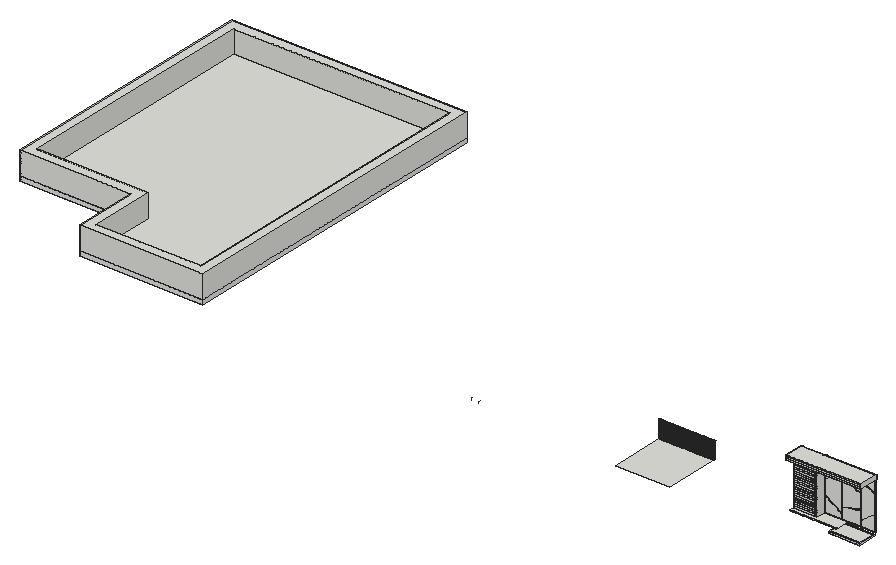
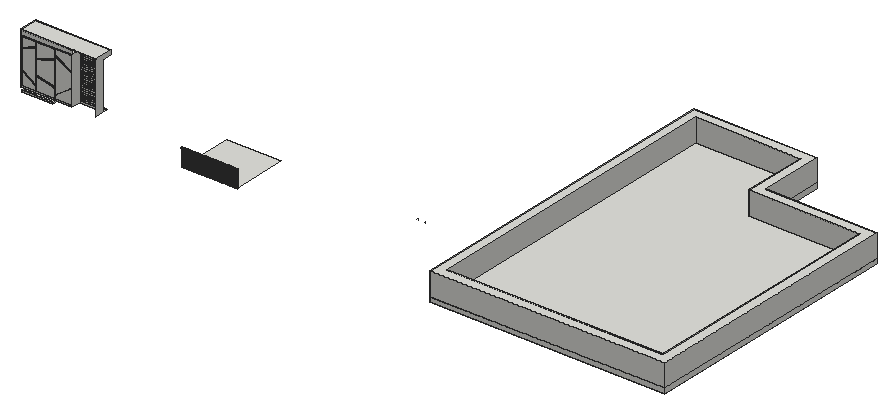
# SketchUp Ruby script. Lengths in inches.
U = 1.inch
M = Sketchup.active_model
def pt(a) = Geom::Point3d.new(a.map { |v| v * U })
def face(e, loops, mat)
  f = e.add_face(loops[0].map { |a| pt(a) })
  loops[1..].each { |l| e.add_face(l.map { |a| pt(a) }).erase! }
  f.material = f.back_material = mat if mat
  f
end
# faces: each face lists its corners as indices into pts; further lists are holes
def faces(e, pts, list, mat = nil) = list.each { |f| face(e, (f[0].is_a?(Array) ? f : [f]).map { |l| l.map { |i| pts[i] } }, mat) }
# xy, xz, yz: faces in a plane at the given z, y or x. An outline is a flat list of corners, or four numbers for a rectangle; further outlines are holes
def ring(l) = l.size == 4 ? [[l[0], l[1]], [l[2], l[1]], [l[2], l[3]], [l[0], l[3]]] : l.each_slice(2).to_a
def flat(e, list, mat, &to3) = list.each { |f| face(e, (f[0].is_a?(Array) ? f : [f]).map { |l| ring(l).map { |u, v| to3.(u, v) } }, mat) }
def xy(e, z, list, mat = nil) = flat(e, list, mat) { |x, y| [x, y, z] }
def xz(e, y, list, mat = nil) = flat(e, list, mat) { |x, z| [x, y, z] }
def yz(e, x, list, mat = nil) = flat(e, list, mat) { |y, z| [x, y, z] }
def lines(e, pts, list) = list.each { |a, b| e.add_line(pt(pts[a]), pt(pts[b])) }
# prism: a flat outline (further loops are holes) pulled along v
def prism(e, loops, v, mat = nil)
  f = face(e, loops, mat); d = Geom::Vector3d.new(v.map { |x| x * U })
  f.pushpull(f.normal.samedirection?(d) ? d.length : -d.length)
end
def box(e, o, s, mat = nil) = prism(e, [[o, [o[0] + s[0], o[1], o[2]], [o[0] + s[0], o[1] + s[1], o[2]], [o[0], o[1] + s[1], o[2]]]], [0, 0, s[2]], mat)
def at(x, y, z, deg = 0) = Geom::Transformation.translation(pt([x, y, z])) * Geom::Transformation.rotation(ORIGIN, Z_AXIS, deg.degrees)
def axes(o, x, y, z) = Geom::Transformation.new([*x, 0, *y, 0, *z, 0, *pt(o).to_a, 1])
def part(name) = M.definitions.add(name)
# library, detail: a bought-in or finely detailed component or shape, given as its bounding box
def library(name, o, s) = part(name).tap { |d| box(d.entities, o, s) }
def detail(e, o, s) = box(e.add_group.entities, o, s)
def put(e, d, t, mat = nil) = e.add_instance(d, t).tap { |i| i.material = mat if mat }
def group(e, t, mat = nil) = e.add_group.tap { |g| g.transformation = t; g.material = mat if mat }.entities
root = M.entities
xy(root,13.08,[[971.17,172.59,1011.17,196.59]])
xy(root,14,[[719.98,146.23,789.98,216.23],[718.98,216.23,719.98,216.73],[719.98,216.23,720.98,216.73],[721.48,216.23,722.48,216.73],[722.48,216.23,723.48,216.73],
  [723.98,216.23,724.98,216.73],[724.98,216.23,725.98,216.73],[726.48,216.23,727.48,216.73],[727.48,216.23,728.48,216.73],[728.98,216.23,729.98,216.73],
  [729.98,216.23,730.98,216.73],[731.48,216.23,732.48,216.73],[732.48,216.23,733.48,216.73],[733.98,216.23,734.98,216.73],[734.98,216.23,735.98,216.73],
  [736.48,216.23,737.48,216.73],[737.48,216.23,738.48,216.73],[738.98,216.23,739.98,216.73],[739.98,216.23,740.98,216.73],[741.48,216.23,742.48,216.73],
  [742.48,216.23,743.48,216.73],[743.98,216.23,744.98,216.73],[744.98,216.23,745.98,216.73],[746.48,216.23,747.48,216.73],[747.48,216.23,748.48,216.73],
  [748.98,216.23,749.98,216.73],[749.98,216.23,750.98,216.73],[751.48,216.23,752.48,216.73],[752.48,216.23,753.48,216.73],[753.98,216.23,754.98,216.73],
  [754.98,216.23,755.98,216.73],[756.48,216.23,757.48,216.73],[757.48,216.23,758.48,216.73],[758.98,216.23,759.98,216.73],[759.98,216.23,760.98,216.73],
  [761.48,216.23,762.48,216.73],[762.48,216.23,763.48,216.73],[763.98,216.23,764.98,216.73],[764.98,216.23,765.98,216.73],[766.48,216.23,767.48,216.73],
  [767.48,216.23,768.48,216.73],[768.98,216.23,769.98,216.73],[769.98,216.23,770.98,216.73],[771.48,216.23,772.48,216.73],[772.48,216.23,773.48,216.73],
  [773.98,216.23,774.98,216.73],[774.98,216.23,775.98,216.73],[776.48,216.23,777.48,216.73],[777.48,216.23,778.48,216.73],[778.98,216.23,779.98,216.73],
  [779.98,216.23,780.98,216.73],[781.48,216.23,782.48,216.73],[782.48,216.23,783.48,216.73],[783.98,216.23,784.98,216.73],[784.98,216.23,785.98,216.73],
  [786.48,216.23,787.48,216.73],[787.48,216.23,788.48,216.73],[788.98,216.23,789.98,216.73],[789.98,216.23,790.98,216.73]])
xy(root,15.08,[[[971.17,172.59,1011.17,196.59],[972.05,173.47,1010.3,195.72]],[972.05,173.47,1010.3,195.72]])
xy(root,18,[[917.17,178.09,919.17,178.59],[919.67,178.09,921.67,178.59],[922.17,178.09,924.17,178.59],[924.67,178.09,926.67,178.59],[927.17,178.09,929.17,178.59],
  [929.67,178.09,931.67,178.59],[932.17,178.09,934.17,178.59],[934.67,178.09,936.67,178.59],[937.17,178.09,939.17,178.59],[939.67,178.09,941.67,178.59],
  [942.17,178.09,944.17,178.59],[944.67,178.09,946.67,178.59],[947.17,178.09,949.17,178.59],[949.67,178.09,951.67,178.59],[952.17,178.09,954.17,178.59],
  [954.67,178.09,956.67,178.59],[957.17,178.09,959.17,178.59],[959.67,178.09,961.67,178.59],[962.17,178.09,964.17,178.59],[964.67,178.09,966.67,178.59],
  [967.17,178.09,969.17,178.59],[969.67,178.09,971.67,178.59],[972.17,178.09,974.17,178.59],[974.67,178.09,976.67,178.59],[917.17,178.59,977.17,178.59,977.17,196.09,947.17,196.09,947.17,184.09,917.17,184.09],
  [917.17,184.09,947.17,184.59]])
xy(root,19,[[994.17,195.59,1012.17,196.09],[948.17,195.72,969.17,196.09],[969.67,195.72,977.17,196.09],[977.17,195.72,993.67,196.09]])
xy(root,20,[[917.17,184.09,947.17,184.59]])
xy(root,20.5,[[917.17,184.09,947.17,184.59]])
xy(root,22.5,[[917.17,184.09,947.17,184.59]])
xy(root,23,[[917.17,184.09,947.17,184.59]])
xy(root,25,[[917.17,184.09,947.17,184.59]])
xy(root,25.5,[[917.17,184.09,947.17,184.59]])
xy(root,27.5,[[917.17,184.09,947.17,184.59]])
xy(root,28,[[917.17,184.09,947.17,184.59]])
xy(root,30,[[917.17,184.09,947.17,184.59]])
xy(root,30.5,[[917.17,184.09,947.17,184.59]])
xy(root,32.5,[[917.17,184.09,947.17,184.59]])
xy(root,33,[[917.17,184.09,947.17,184.59]])
xy(root,35,[[917.17,184.09,947.17,184.59]])
xy(root,35.5,[[917.17,184.09,947.17,184.59]])
xy(root,36,[[718.98,216.23,720.98,216.73],[721.48,216.23,723.48,216.73],[723.98,216.23,725.98,216.73],[726.48,216.23,728.48,216.73],[728.98,216.23,730.98,216.73],
  [731.48,216.23,733.48,216.73],[733.98,216.23,735.98,216.73],[736.48,216.23,738.48,216.73],[738.98,216.23,740.98,216.73],[741.48,216.23,743.48,216.73],
  [743.98,216.23,745.98,216.73],[746.48,216.23,748.48,216.73],[748.98,216.23,750.98,216.73],[751.48,216.23,753.48,216.73],[753.98,216.23,755.98,216.73],
  [756.48,216.23,758.48,216.73],[758.98,216.23,760.98,216.73],[761.48,216.23,763.48,216.73],[763.98,216.23,765.98,216.73],[766.48,216.23,768.48,216.73],
  [768.98,216.23,770.98,216.73],[771.48,216.23,773.48,216.73],[773.98,216.23,775.98,216.73],[776.48,216.23,778.48,216.73],[778.98,216.23,780.98,216.73],
  [781.48,216.23,783.48,216.73],[783.98,216.23,785.98,216.73],[786.48,216.23,788.48,216.73],[788.98,216.23,790.98,216.73],[718.98,216.73,790.98,217.23]])
xy(root,37.5,[[917.17,184.09,947.17,184.59]])
xy(root,38,[[917.17,184.09,947.17,184.59]])
xy(root,40,[[917.17,184.09,947.17,184.59]])
xy(root,40.5,[[917.17,184.09,947.17,184.59]])
xy(root,42.5,[[917.17,184.09,947.17,184.59]])
xy(root,43,[[917.17,184.09,947.17,184.59]])
xy(root,45,[[917.17,184.09,947.17,184.59]])
xy(root,45.5,[[917.17,184.09,947.17,184.59]])
xy(root,47.5,[[917.17,184.09,947.17,184.59]])
xy(root,48,[[917.17,184.09,947.17,184.59]])
xy(root,50,[[917.17,184.09,947.17,184.59]])
xy(root,50.5,[[917.17,184.09,947.17,184.59]])
xy(root,52.5,[[917.17,184.09,947.17,184.59]])
xy(root,53,[[917.17,184.09,947.17,184.59]])
xy(root,55,[[917.17,184.09,947.17,184.59]])
xy(root,55.5,[[917.17,184.09,947.17,184.59]])
xy(root,57.5,[[917.17,184.09,947.17,184.59]])
xy(root,58,[[917.17,184.09,947.17,184.59]])
xy(root,60,[[917.17,184.09,947.17,184.59]])
xy(root,60.5,[[917.17,184.09,947.17,184.59]])
xy(root,62.5,[[917.17,184.09,947.17,184.59]])
xy(root,63,[[917.17,184.09,947.17,184.59]])
xy(root,65,[[917.17,184.09,947.17,184.59]])
xy(root,65.5,[[917.17,184.09,947.17,184.59]])
xy(root,67.5,[[917.17,184.09,947.17,184.59]])
xy(root,68,[[917.17,184.09,947.17,184.59]])
xy(root,70,[[917.17,184.09,947.17,184.59]])
xy(root,70.5,[[917.17,184.09,947.17,184.59]])
xy(root,72.5,[[917.17,184.09,947.17,184.59]])
xy(root,73,[[917.17,184.09,947.17,184.59]])
xy(root,75,[[917.17,184.09,947.17,184.59]])
xy(root,75.5,[[917.17,184.09,947.17,184.59]])
xy(root,77,[[994.17,195.59,1012.17,196.09],[948.17,195.72,969.17,196.09],[969.67,195.72,993.67,196.09]])
xy(root,77.5,[[917.17,184.09,947.17,184.59]])
xy(root,78,[[917.17,172.59,917.17,184.59,947.17,184.59,947.17,196.09,1013.17,196.09,1011.17,172.59],[1011.17,172.59,1013.17,196.09,1013.17,172.59]])
xy(root,84,[[917.17,172.59,1013.17,196.09],[917.17,196.09,947.17,196.59],[947.17,196.09,1013.17,196.59]])
xz(root,172.59,[[[971.17,13.08,1011.17,15.08],[971.67,13.58,1010.67,14.58]],[971.67,13.58,1010.67,14.58],[[917.17,78,1013.17,84],[918.17,79,1012.17,83]],[918.17,79,1012.17,83]])
xz(root,184.09,[[917.17,18,947.17,20],[917.17,20.5,947.17,22.5],[917.17,23,947.17,25],[917.17,25.5,947.17,27.5],[917.17,28,947.17,30],
  [917.17,30.5,947.17,32.5],[917.17,33,947.17,35],[917.17,35.5,947.17,37.5],[917.17,38,947.17,40],[917.17,40.5,947.17,42.5],
  [917.17,43,947.17,45],[917.17,45.5,947.17,47.5],[917.17,48,947.17,50],[917.17,50.5,947.17,52.5],[917.17,53,947.17,55],
  [917.17,55.5,947.17,57.5],[917.17,58,947.17,60],[917.17,60.5,947.17,62.5],[917.17,63,947.17,65],[917.17,65.5,947.17,67.5],
  [917.17,68,947.17,70],[917.17,70.5,947.17,72.5],[917.17,73,947.17,75],[917.17,75.5,947.17,77.5]])
xz(root,184.59,[[917.17,18,947.17,20],[917.17,20,947.17,20.5],[917.17,20.5,947.17,22.5],[917.17,22.5,947.17,23],[917.17,23,947.17,25],
  [917.17,25,947.17,25.5],[917.17,25.5,947.17,27.5],[917.17,27.5,947.17,28],[917.17,28,947.17,30],[917.17,30,947.17,30.5],
  [917.17,30.5,947.17,32.5],[917.17,32.5,947.17,33],[917.17,33,947.17,35],[917.17,35,947.17,35.5],[917.17,35.5,947.17,37.5],
  [917.17,37.5,947.17,38],[917.17,38,947.17,40],[917.17,40,947.17,40.5],[917.17,40.5,947.17,42.5],[917.17,42.5,947.17,43],
  [917.17,43,947.17,45],[917.17,45,947.17,45.5],[917.17,45.5,947.17,47.5],[917.17,47.5,947.17,48],[917.17,48,947.17,50],
  [917.17,50,947.17,50.5],[917.17,50.5,947.17,52.5],[917.17,52.5,947.17,53],[917.17,53,947.17,55],[917.17,55,947.17,55.5],
  [917.17,55.5,947.17,57.5],[917.17,57.5,947.17,58],[917.17,58,947.17,60],[917.17,60,947.17,60.5],[917.17,60.5,947.17,62.5],
  [917.17,62.5,947.17,63],[917.17,63,947.17,65],[917.17,65,947.17,65.5],[917.17,65.5,947.17,67.5],[917.17,67.5,947.17,68],
  [917.17,68,947.17,70],[917.17,70,947.17,70.5],[917.17,70.5,947.17,72.5],[917.17,72.5,947.17,73],[917.17,73,947.17,75],
  [917.17,75,947.17,75.5],[917.17,75.5,947.17,77.5],[917.17,77.5,947.17,78]])
xz(root,195.59,[[994.17,19,1012.17,19,1012.17,37.79,994.17,25.79],[994.17,26.39,1012.17,38.39,1012.17,62.76,994.17,70.87],[1012.17,63.3125,1012.17,77,994.17,77,994.17,71.42]])
xz(root,195.72,[[948.17,19,969.17,19,969.17,23.8,948.17,38.21],[969.67,19,993.67,19,993.67,37.88,969.67,32.37],[969.17,24.4,969.17,69.42,948.17,56.84,948.17,38.82],[969.67,32.88,993.67,38.39,993.67,55.9,969.67,65.8],[993.67,56.44,993.67,77,969.67,77,969.67,66.34],
  [948.17,57.42,969.17,70.01,969.17,77,948.17,77]])
xz(root,196.09,[[[947.17,18,1013.17,78],[948.17,19,1012.17,77]],[969.17,19,969.67,77],[993.67,19,994.17,77],[969.17,23.8,969.17,24.4,948.17,38.82,948.17,38.21],[994.17,25.79,1012.17,37.79,1012.17,38.39,994.17,26.39],
  [969.67,32.37,993.67,37.88,993.67,38.39,969.67,32.88],[993.67,55.9,993.67,56.44,969.67,66.34,969.67,65.8],[948.17,56.84,969.17,69.42,969.17,70.01,948.17,57.42],[1012.17,62.76,1012.17,63.3125,994.17,71.42,994.17,70.87],[947.17,78,1013.17,84]])
xz(root,196.59,[[971.17,13.08,1011.17,15.08]])
xz(root,216.23,[[718.98,14,720.98,36],[721.48,14,723.48,36],[723.98,14,725.98,36],[726.48,14,728.48,36],[728.98,14,730.98,36],
  [731.48,14,733.48,36],[733.98,14,735.98,36],[736.48,14,738.48,36],[738.98,14,740.98,36],[741.48,14,743.48,36],
  [743.98,14,745.98,36],[746.48,14,748.48,36],[748.98,14,750.98,36],[751.48,14,753.48,36],[753.98,14,755.98,36],
  [756.48,14,758.48,36],[758.98,14,760.98,36],[761.48,14,763.48,36],[763.98,14,765.98,36],[766.48,14,768.48,36],
  [768.98,14,770.98,36],[771.48,14,773.48,36],[773.98,14,775.98,36],[776.48,14,778.48,36],[778.98,14,780.98,36],
  [781.48,14,783.48,36],[783.98,14,785.98,36],[786.48,14,788.48,36],[788.98,14,790.98,36]])
xz(root,216.73,[[718.98,14,720.98,36],[721.48,14,723.48,36],[723.98,14,725.98,36],[726.48,14,728.48,36],[728.98,14,730.98,36],
  [731.48,14,733.48,36],[733.98,14,735.98,36],[736.48,14,738.48,36],[738.98,14,740.98,36],[741.48,14,743.48,36],
  [743.98,14,745.98,36],[746.48,14,748.48,36],[748.98,14,750.98,36],[751.48,14,753.48,36],[753.98,14,755.98,36],
  [756.48,14,758.48,36],[758.98,14,760.98,36],[761.48,14,763.48,36],[763.98,14,765.98,36],[766.48,14,768.48,36],
  [768.98,14,770.98,36],[771.48,14,773.48,36],[773.98,14,775.98,36],[776.48,14,778.48,36],[778.98,14,780.98,36],
  [781.48,14,783.48,36],[783.98,14,785.98,36],[786.48,14,788.48,36],[788.98,14,790.98,36]])
yz(root,718.98,[[216.23,14,216.73,36]])
yz(root,720.98,[[216.23,14,216.73,36]])
yz(root,721.48,[[216.23,14,216.73,36]])
yz(root,723.48,[[216.23,14,216.73,36]])
yz(root,723.98,[[216.23,14,216.73,36]])
yz(root,725.98,[[216.23,14,216.73,36]])
yz(root,726.48,[[216.23,14,216.73,36]])
yz(root,728.48,[[216.23,14,216.73,36]])
yz(root,728.98,[[216.23,14,216.73,36]])
yz(root,730.98,[[216.23,14,216.73,36]])
yz(root,731.48,[[216.23,14,216.73,36]])
yz(root,733.48,[[216.23,14,216.73,36]])
yz(root,733.98,[[216.23,14,216.73,36]])
yz(root,735.98,[[216.23,14,216.73,36]])
yz(root,736.48,[[216.23,14,216.73,36]])
yz(root,738.48,[[216.23,14,216.73,36]])
yz(root,738.98,[[216.23,14,216.73,36]])
yz(root,740.98,[[216.23,14,216.73,36]])
yz(root,741.48,[[216.23,14,216.73,36]])
yz(root,743.48,[[216.23,14,216.73,36]])
yz(root,743.98,[[216.23,14,216.73,36]])
yz(root,745.98,[[216.23,14,216.73,36]])
yz(root,746.48,[[216.23,14,216.73,36]])
yz(root,748.48,[[216.23,14,216.73,36]])
yz(root,748.98,[[216.23,14,216.73,36]])
yz(root,750.98,[[216.23,14,216.73,36]])
yz(root,751.48,[[216.23,14,216.73,36]])
yz(root,753.48,[[216.23,14,216.73,36]])
yz(root,753.98,[[216.23,14,216.73,36]])
yz(root,755.98,[[216.23,14,216.73,36]])
yz(root,756.48,[[216.23,14,216.73,36]])
yz(root,758.48,[[216.23,14,216.73,36]])
yz(root,758.98,[[216.23,14,216.73,36]])
yz(root,760.98,[[216.23,14,216.73,36]])
yz(root,761.48,[[216.23,14,216.73,36]])
yz(root,763.48,[[216.23,14,216.73,36]])
yz(root,763.98,[[216.23,14,216.73,36]])
yz(root,765.98,[[216.23,14,216.73,36]])
yz(root,766.48,[[216.23,14,216.73,36]])
yz(root,768.48,[[216.23,14,216.73,36]])
yz(root,768.98,[[216.23,14,216.73,36]])
yz(root,770.98,[[216.23,14,216.73,36]])
yz(root,771.48,[[216.23,14,216.73,36]])
yz(root,773.48,[[216.23,14,216.73,36]])
yz(root,773.98,[[216.23,14,216.73,36]])
yz(root,775.98,[[216.23,14,216.73,36]])
yz(root,776.48,[[216.23,14,216.73,36]])
yz(root,778.48,[[216.23,14,216.73,36]])
yz(root,778.98,[[216.23,14,216.73,36]])
yz(root,780.98,[[216.23,14,216.73,36]])
yz(root,781.48,[[216.23,14,216.73,36]])
yz(root,783.48,[[216.23,14,216.73,36]])
yz(root,783.98,[[216.23,14,216.73,36]])
yz(root,785.98,[[216.23,14,216.73,36]])
yz(root,786.48,[[216.23,14,216.73,36]])
yz(root,788.48,[[216.23,14,216.73,36]])
yz(root,788.98,[[216.23,14,216.73,36]])
yz(root,790.98,[[216.23,14,216.73,36]])
yz(root,917.17,[[184.59,18,184.59,78,172.59,78,172.59,84,196.09,84,196.09,18],[184.09,18,184.59,20],[196.09,18,196.59,84],[184.09,20.5,184.59,22.5],[184.09,23,184.59,25],
  [184.09,25.5,184.59,27.5],[184.09,28,184.59,30],[184.09,30.5,184.59,32.5],[184.09,33,184.59,35],[184.09,35.5,184.59,37.5],
  [184.09,38,184.59,40],[184.09,40.5,184.59,42.5],[184.09,43,184.59,45],[184.09,45.5,184.59,47.5],[184.09,48,184.59,50],
  [184.09,50.5,184.59,52.5],[184.09,53,184.59,55],[184.09,55.5,184.59,57.5],[184.09,58,184.59,60],[184.09,60.5,184.59,62.5],
  [184.09,63,184.59,65],[184.09,65.5,184.59,67.5],[184.09,68,184.59,70],[184.09,70.5,184.59,72.5],[184.09,73,184.59,75],
  [184.09,75.5,184.59,77.5]])
yz(root,947.17,[[184.09,18,184.59,20],[184.59,18,196.09,78],[184.09,20.5,184.59,22.5],[184.09,23,184.59,25],[184.09,25.5,184.59,27.5],
  [184.09,28,184.59,30],[184.09,30.5,184.59,32.5],[184.09,33,184.59,35],[184.09,35.5,184.59,37.5],[184.09,38,184.59,40],
  [184.09,40.5,184.59,42.5],[184.09,43,184.59,45],[184.09,45.5,184.59,47.5],[184.09,48,184.59,50],[184.09,50.5,184.59,52.5],
  [184.09,53,184.59,55],[184.09,55.5,184.59,57.5],[184.09,58,184.59,60],[184.09,60.5,184.59,62.5],[184.09,63,184.59,65],
  [184.09,65.5,184.59,67.5],[184.09,68,184.59,70],[184.09,70.5,184.59,72.5],[184.09,73,184.59,75],[184.09,75.5,184.59,77.5]])
yz(root,948.17,[[195.72,19,196.09,38.21],[195.72,38.82,196.09,56.84],[195.72,57.42,196.09,77]])
yz(root,969.17,[[195.72,19,196.09,23.8],[195.72,24.4,196.09,69.42],[195.72,70.01,196.09,77]])
yz(root,969.67,[[195.72,19,196.09,32.37],[195.72,32.88,196.09,65.8],[195.72,66.34,196.09,77]])
yz(root,971.17,[[172.59,13.08,196.59,15.08]])
yz(root,993.67,[[195.72,19,196.09,37.88],[195.72,38.39,196.09,55.9],[195.72,56.44,196.09,77]])
yz(root,994.17,[[195.59,19,196.09,25.79],[195.59,26.39,196.09,70.87],[195.59,71.42,196.09,77]])
yz(root,1011.17,[[172.59,13.08,196.59,15.08]])
yz(root,1012.17,[[195.59,19,196.09,37.79],[195.59,38.39,196.09,62.76],[195.59,63.3125,196.09,77]])
yz(root,1013.17,[[172.59,78,196.09,84],[196.09,78,196.59,84]])
p = [[969.17,196.09,23.8],[948.17,196.09,38.21],[948.17,195.72,38.21],[969.17,195.72,23.8],[948.17,196.09,38.82],[969.17,196.09,24.4],
  [969.17,195.72,24.4],[948.17,195.72,38.82],[1012.17,196.09,37.79],[994.17,196.09,25.79],[994.17,195.59,25.79],[1012.17,195.59,37.79],
  [994.17,196.09,26.39],[1012.17,196.09,38.39],[1012.17,195.59,38.39],[994.17,195.59,26.39],[993.67,196.09,37.88],[969.67,196.09,32.37],
  [969.67,195.72,32.37],[993.67,195.72,37.88],[969.67,196.09,32.88],[993.67,196.09,38.39],[993.67,195.72,38.39],[969.67,195.72,32.88],
  [993.67,196.09,55.9],[969.67,196.09,65.8],[969.67,195.72,65.8],[993.67,195.72,55.9],[969.67,196.09,66.34],[993.67,196.09,56.44],
  [993.67,195.72,56.44],[969.67,195.72,66.34],[969.17,196.09,69.42],[948.17,196.09,56.84],[948.17,195.72,56.84],[969.17,195.72,69.42],
  [948.17,196.09,57.42],[969.17,196.09,70.01],[969.17,195.72,70.01],[948.17,195.72,57.42],[1012.17,196.09,62.76],[994.17,196.09,70.87],
  [994.17,195.59,70.87],[1012.17,195.59,62.76],[994.17,196.09,71.42],[1012.17,196.09,63.3125],[1012.17,195.59,63.3125],[994.17,195.59,71.42],
  [536.43,159.5,18],[536.43,157.5,18],[526.43,159.5,18],[526.43,157.5,18],[526.43,157.5,16],[536.43,157.5,16]]
faces(root,p,[[0,1,2,3],[4,5,6,7],[8,9,10,11],[12,13,14,15],[16,17,18,19],[20,21,22,23],[24,25,26,27],[28,29,30,31],
  [32,33,34,35],[36,37,38,39],[40,41,42,43],[44,45,46,47]])
lines(root,p,[[48,49],[50,51],[52,51],[53,49]])
g1 = group(root,at(10.33,82.68,118.11))
prism(g1,[[[0,0,0],[0,338.58,0],[299.21,338.58,0],[299.21,-82.68,0],[141.73,-82.68,0],[141.73,0,0]]],[0,0,5.91])
g2 = group(root,at(10.33,82.68,124.02))
prism(g2,[[[0,0,0],[0,338.58,0],[299.21,338.58,0],[299.21,-82.68,0],[141.73,-82.68,0],[141.73,0,0]],[[287.4,-70.87,0],[287.4,326.77,0],[11.8125,326.77,0],[11.8125,11.8125,0],[153.54,11.8125,0],[153.54,-70.87,0]]],[0,0,29.53])
